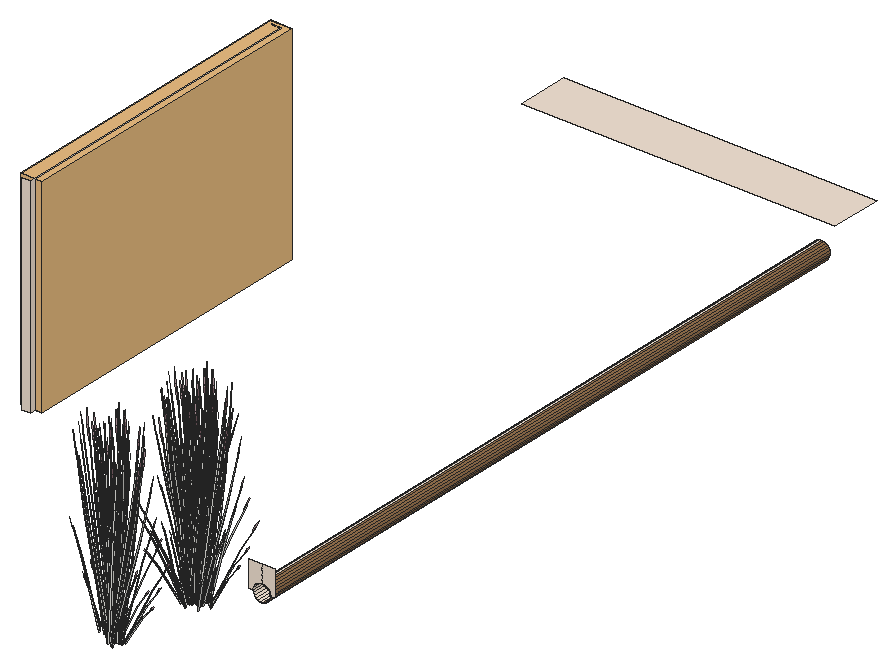
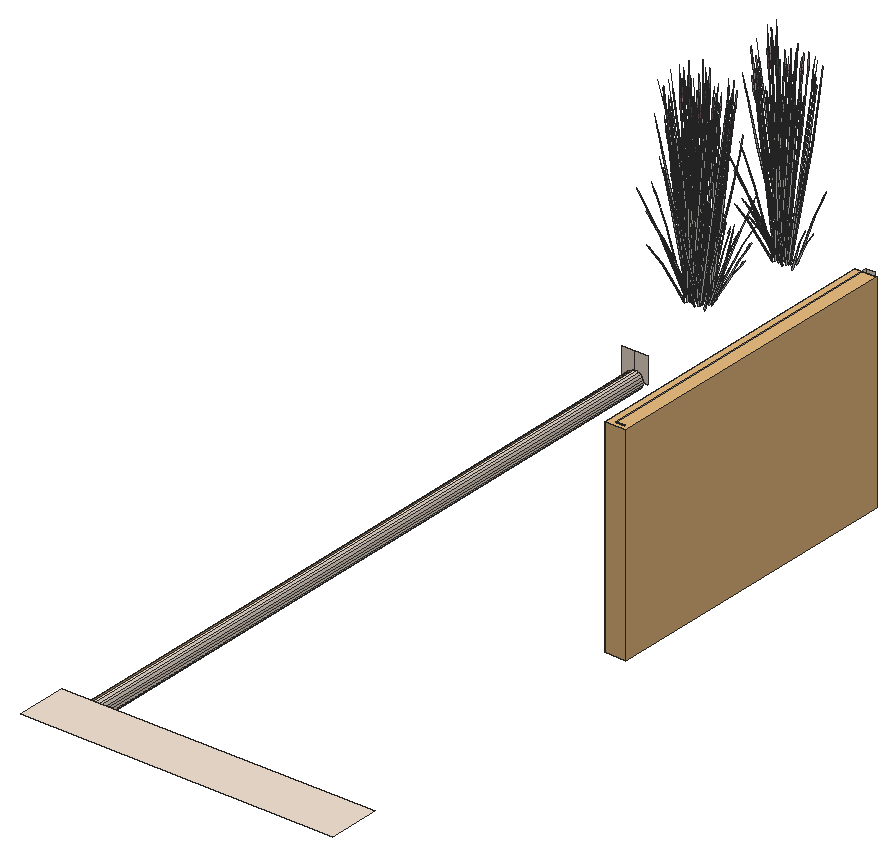
# SketchUp Ruby script. Lengths in inches.
U = 1.inch
M = Sketchup.active_model
def pt(a) = Geom::Point3d.new(a.map { |v| v * U })
def face(e, loops, mat)
  f = e.add_face(loops[0].map { |a| pt(a) })
  loops[1..].each { |l| e.add_face(l.map { |a| pt(a) }).erase! }
  f.material = f.back_material = mat if mat
  f
end
# faces: each face lists its corners as indices into pts; further lists are holes
def faces(e, pts, list, mat = nil) = list.each { |f| face(e, (f[0].is_a?(Array) ? f : [f]).map { |l| l.map { |i| pts[i] } }, mat) }
# xy, xz, yz: faces in a plane at the given z, y or x. An outline is a flat list of corners, or four numbers for a rectangle; further outlines are holes
def ring(l) = l.size == 4 ? [[l[0], l[1]], [l[2], l[1]], [l[2], l[3]], [l[0], l[3]]] : l.each_slice(2).to_a
def flat(e, list, mat, &to3) = list.each { |f| face(e, (f[0].is_a?(Array) ? f : [f]).map { |l| ring(l).map { |u, v| to3.(u, v) } }, mat) }
def xy(e, z, list, mat = nil) = flat(e, list, mat) { |x, y| [x, y, z] }
def xz(e, y, list, mat = nil) = flat(e, list, mat) { |x, z| [x, y, z] }
def yz(e, x, list, mat = nil) = flat(e, list, mat) { |y, z| [x, y, z] }
def lines(e, pts, list) = list.each { |a, b| e.add_line(pt(pts[a]), pt(pts[b])) }
# prism: a flat outline (further loops are holes) pulled along v
def prism(e, loops, v, mat = nil)
  f = face(e, loops, mat); d = Geom::Vector3d.new(v.map { |x| x * U })
  f.pushpull(f.normal.samedirection?(d) ? d.length : -d.length)
end
def box(e, o, s, mat = nil) = prism(e, [[o, [o[0] + s[0], o[1], o[2]], [o[0] + s[0], o[1] + s[1], o[2]], [o[0], o[1] + s[1], o[2]]]], [0, 0, s[2]], mat)
def at(x, y, z, deg = 0) = Geom::Transformation.translation(pt([x, y, z])) * Geom::Transformation.rotation(ORIGIN, Z_AXIS, deg.degrees)
def axes(o, x, y, z) = Geom::Transformation.new([*x, 0, *y, 0, *z, 0, *pt(o).to_a, 1])
def part(name) = M.definitions.add(name)
# library, detail: a bought-in or finely detailed component or shape, given as its bounding box
def library(name, o, s) = part(name).tap { |d| box(d.entities, o, s) }
def detail(e, o, s) = box(e.add_group.entities, o, s)
def put(e, d, t, mat = nil) = e.add_instance(d, t).tap { |i| i.material = mat if mat }
def group(e, t, mat = nil) = e.add_group.tap { |g| g.transformation = t; g.material = mat if mat }.entities
root = M.entities
M.materials.add("C01_Vanilla_Cream").color = [244, 228, 212]
M.materials.add("LightPink_Translucent").color = [144, 107, 117]
M.materials["LightPink_Translucent"].alpha = 0.75
M.materials.add("Wood_Floor_01_1K").color = [146, 111, 76]
c1 = part("blade")
p = [[2.15,0.21,22],[0,0.17,0],[0.09,0.45,0],[2.18,0.31,22],[2.29,0.31,22],[0.38,0.45,0],
  [2.48,0.24,33],[2.49,0.24,33],[2.48,0.22,33]]
faces(c1.entities,p,[[0,1,2,3],[4,5,2,3],[6,3,4,7],[8,0,3,6]])
c2 = part("seeds")
p = [[0.3,-0.1,1.38],[-0.01,-0.03,1.59],[-0.01,-0.03,0.03],[0.14,-0.07,-0.07],[0.29,-0.03,3],[0.15,0.01,3.11]]
faces(c2.entities,p,[[0,1,2,3],[1,0,4,5]],"LightPink_Translucent")
c3 = part("blade with seeds")
put(c3.entities,c1,at(0,0,0))
put(c3.entities,c2,axes([2.4,0.25,30.99],[1.5799,-0.05474,1.17369],[-0.12525,1.92788,0.29478],[-0.07173,-0.02425,1.56792]))
c4 = library("Double casement window",[0,0,0],[5.02,56.42,60])
xy(root,498,[[288,324,290,396],[288,468,360,480]],"C01_Vanilla_Cream")
xz(root,306.76,[[354,492,354,498,357,498,357,494,356.48,493.93,356,493.73,355.59,493.41,355.27,493,355.07,492.52,355,492],[359,492,358.93,492.52,358.73,493,358.41,493.41,358,493.73,357.52,493.93,357,494,357,498,360,498,360,492]],"C01_Vanilla_Cream")
xz(root,324,[[288,498,290,546]],"C01_Vanilla_Cream")
xz(root,396,[[288,498,290,546]],"C01_Vanilla_Cream")
yz(root,290,[[[324,498,396,546],[327,501,358.5,543],[361.5,501,393,543]]],"C01_Vanilla_Cream")
p = [[357,306.76,490],[356.48,306.76,490.07],[356.48,468,490.07],[357,468,490],[357.52,306.76,490.07],[357.52,468,490.07],
  [356,306.76,490.27],[356,468,490.27],[358,306.76,490.27],[358,468,490.27],[355.59,306.76,490.59],[355.59,468,490.59],
  [358.41,306.76,490.59],[358.41,468,490.59],[355.27,306.76,491],[355.27,468,491],[358.73,306.76,491],[358.73,468,491],
  [355.07,306.76,491.48],[355.07,468,491.48],[358.93,306.76,491.48],[358.93,468,491.48],[355,306.76,492],[355,468,492],
  [359,306.76,492],[359,468,492],[355.07,306.76,492.52],[355.07,468,492.52],[358.93,306.76,492.52],[358.93,468,492.52],
  [355.27,306.76,493],[355.27,468,493],[358.73,306.76,493],[358.73,468,493],[355.59,306.76,493.41],[355.59,468,493.41],
  [358.41,306.76,493.41],[358.41,468,493.41],[356,306.76,493.73],[356,468,493.73],[358,306.76,493.73],[358,468,493.73],
  [356.48,306.76,493.93],[356.48,468,493.93],[357.52,306.76,493.93],[357.52,468,493.93],[357,306.76,494],[357,468,494]]
faces(root,p,[[0,1,2,3],[1,6,7,2],[6,10,11,7],[10,14,15,11],[14,18,19,15],[18,22,23,19],[22,26,27,23],[26,30,31,27],
  [30,34,35,31],[34,38,39,35],[38,42,43,39],[42,46,47,43]],"C01_Vanilla_Cream")
faces(root,p,[[4,0,3,5],[8,4,5,9],[12,8,9,13],[16,12,13,17],[20,16,17,21],[24,20,21,25],[28,24,25,29],[32,28,29,33],
  [36,32,33,37],[40,36,37,41],[44,40,41,45],[46,44,45,47]],"Wood_Floor_01_1K")
put(root,c3,axes([353.44,266.61,499.52],[-0.13078,-0.42928,-0.23233],[0.51941,-0.1219,0.23233],[-0.10471,-0.0495,1.0423]))
put(root,c3,axes([354.11,266.59,499.86],[0.59825,-0.13076,0.13232],[0.14773,0.48663,0.26315],[-0.05336,-0.0709,1.20305]))
put(root,c3,axes([355.34,264.75,500],[0.56211,-0.32708,-0.21822],[0.3738,0.46216,-0.37502],[0.13869,0.04694,1.19781]))
put(root,c3,axes([353.3,266.8,499.51],[-0.52105,-0.24633,-0.37238],[0.31144,-0.44171,0],[-0.11867,-0.0561,1.18128]))
put(root,c3,axes([356.76,263.88,499.51],[0.52105,0.24633,-0.37238],[-0.31144,0.44171,0],[0.11867,0.0561,1.18128]))
put(root,c3,axes([355.77,265.28,499.65],[0.62289,0,0],[0,0.51004,0],[0,0,1.33805]))
put(root,c3,axes([354.71,265.93,500],[-0.56211,0.32708,-0.21822],[-0.3738,-0.46216,-0.37502],[-0.13869,-0.04694,1.19781]))
put(root,c3,axes([355.95,264.09,499.86],[-0.59825,0.13076,0.13232],[-0.14773,-0.48663,0.26315],[0.05336,0.0709,1.20305]))
put(root,c3,axes([356.61,264.0625,499.52],[0.13078,0.42928,-0.23233],[-0.51941,0.1219,0.23233],[0.10471,0.0495,1.0423]))
put(root,c3,axes([355.57,265.02,499.79],[-0.70367,-0.1038,0.36899],[0.1432,-0.58624,0.1448],[0.10283,0.05661,1.2811]))
put(root,c3,axes([355.01,266.47,499.65],[-0.18165,-0.42474,0],[0.51872,-0.14874,0],[0,0,1.15778]))
put(root,c3,axes([354.66,266.07,499.96],[-0.1074,0.43968,0.1086],[-0.52474,-0.07632,-0.3101],[-0.0955,-0.04515,0.95058]))
put(root,c3,axes([355.6875,266.41,499.64],[0.5845,-0.16716,-0.14398],[0.20539,0.48152,0.00006],[0.06452,-0.01848,1.30423]))
put(root,c3,axes([355.89,266.61,499.86],[0.16083,-0.48962,0.13232],[0.58854,0.13856,0.26315],[-0.10167,0.00238,1.20305]))
put(root,c3,axes([355.76,265.5,499.66],[0.38863,0.31822,0],[-0.38863,0.31822,0],[0,0,1.2695]))
put(root,c3,axes([356.81,265.36,499.86],[-0.43742,-0.35886,0.13232],[0.44081,-0.34807,0.26315],[-0.04831,0.07329,1.20305]))
put(root,c3,axes([356,264.82,499.54],[0.57914,0.08077,-0.46765],[-0.12221,0.49823,-0.12274],[0.17283,0.06037,1.03225]))
put(root,c3,axes([358.56,265.69,500.07],[-0.34399,0.08133,0.86145],[0.16192,-0.33614,0.63294],[0.18249,0.023,0.18974]))
put(root,c3,axes([354.88,266.66,499.65],[-0.56127,-0.22118,0],[0.27012,-0.45959,0],[0,0,1.2203]))
put(root,c3,axes([355.34,266.07,499.85],[-0.54364,-0.39653,-0.18894],[0.45745,-0.44527,0.41347],[-0.14639,0.04639,1.26162]))
put(root,c3,axes([353.91,266.83,499.86],[0.52105,0.24633,0.37238],[-0.31144,0.44171,0],[-0.11867,-0.0561,1.18128]))
put(root,c3,axes([355.75,265.13,500.04],[0.27012,-0.44393,0.33554],[0.56127,0.21365,-0.16149],[0,0.10233,1.07733]))
put(root,c3,axes([355.65,265.38,499.72],[0,0.56976,-0.04228],[-0.69617,0,0],[0,0.01791,1.34526]))
put(root,c3,axes([355.7,264.98,499.66],[0.33445,0.41351,-0.33554],[-0.50659,0.29119,0.16149],[0.10823,0.05117,1.07733]))
put(root,c3,axes([353.61,267.09,499.78],[-0.34808,0.49367,0],[-0.58235,-0.27531,-0.38706],[-0.13264,-0.0627,1.22783]))
put(root,c3,axes([357.17,265.38,499.86],[0,-0.49266,0.37238],[0.62289,0,0],[0,0.11221,1.18128]))
put(root,c3,axes([355.61,265.75,500.04],[0.60457,-0.03041,0.33554],[0.05467,0.50484,-0.16149],[-0.10823,0.05117,1.07733]))
put(root,c3,axes([355.98,265.23,499.96],[0.51872,-0.14368,0.1086],[0.18165,0.41027,-0.3101],[0,0.09029,0.95058]))
put(root,c3,axes([355.07,265.99,499.66],[-0.60457,0.03041,-0.33554],[-0.05467,-0.50484,0.16149],[-0.10823,0.05117,1.07733]))
put(root,c3,axes([357.91,266.23,499.94],[-0.13408,-0.12117,1.07251],[0.17446,-0.40083,-0.23066],[0.27128,0.0543,0.45856]))
put(root,c3,axes([355.52,266.67,499.65],[0.56127,0.22118,0],[-0.27012,0.45959,0],[0,0,1.31215]))
put(root,c3,axes([355.74,267.16,499.64],[-0.34375,-0.4954,-0.03857],[0.58235,-0.27531,0.38706],[-0.1435,0.04717,1.22723]))
put(root,c3,axes([355.62,265.96,499.96],[0.41131,0.296,0.1086],[-0.34309,0.33395,-0.3101],[-0.0955,0.04515,0.95058]))
put(root,c3,axes([356.05,266.875,499.86],[0.52105,-0.24633,0.37238],[0.31144,0.44171,0],[-0.11867,0.0561,1.18128]))
put(root,c3,axes([355.3125,266.49,499.72],[0.24206,0.56598,-0.04509],[-0.69162,0.19832,0],[0.00845,0.01976,1.2913]))
put(root,c3,axes([355.58,267.1,499.52],[-0.51941,-0.1219,-0.23233],[0.13078,-0.42928,0.23233],[-0.10471,0.0495,1.0423]))
put(root,c3,axes([351.83,266.23,499.94],[0.19348,0.04044,1.07251],[0.1247,0.41309,-0.23066],[-0.26282,0.07733,0.45856]))
put(root,c3,axes([357.59,265.46,499.78],[0.69617,0,0],[0,0.55062,-0.38706],[0,0.12541,1.22783]))
put(root,c3,axes([357.3125,265.74,499.65],[-0.69582,-0.00394,-0.03732],[0,-0.55062,0.37457],[-0.02187,0.12535,1.18764]))
put(root,c3,axes([355.81,265.26,500],[0.62699,0.23507,-0.21822],[-0.3019,0.49615,-0.37502],[0.0197,0.12182,1.19781]))
put(root,c3,axes([351.43,267.09,500.07],[0.23202,-0.22328,0.86145],[0.09155,0.35348,0.63294],[-0.16768,0.06329,0.18974]))
put(root,c3,axes([357.17,265.82,499.52],[-0.38863,0.30738,-0.23233],[-0.38863,-0.30738,0.23233],[0,0.09901,1.0423]))
put(root,c3,axes([355.49,265.85,500],[0.06488,0.56215,-0.21822],[-0.6757,0.03399,-0.37502],[-0.11898,0.07488,1.19781]))
put(root,c3,axes([355.74,265.63,499.66],[-0.27012,0.44393,-0.33554],[-0.56127,-0.21365,0.16149],[0,0.10233,1.07733]))
put(root,c3,axes([355.09,266.28,499.54],[-0.375,0.3703,-0.46765],[-0.46584,-0.33578,-0.12274],[-0.15027,0.09237,1.03225]))
put(root,c3,axes([355.75,266.91,499.75],[0.697,0.16013,0.23067],[-0.17437,0.57237,-0.27369],[-0.11536,0.07164,1.23664]))
put(root,c3,axes([355.7,267.29,499.51],[-0.52105,0.24633,-0.37238],[-0.31144,-0.44171,0],[-0.11867,0.0561,1.18128]))
put(root,c3,axes([357.44,265.83,499.51],[0,0.49266,-0.37238],[-0.62289,0,0],[0,0.11221,1.18128]))
put(root,c3,axes([356.64,266.86,500.07],[-0.31347,-0.14166,0.86145],[0.40476,-0.14393,0.63294],[0.10917,0.12192,0.18974]))
put(root,c3,axes([356.18,267.22,499.78],[0.34808,0.49367,0],[-0.58235,0.27531,-0.38706],[-0.13264,0.0627,1.22783]))
put(root,c3,axes([356.73,267.38,499.12],[0.04056,-0.07113,1.32257],[0.51066,-0.20948,-0.20205],[0.15482,0.10842,0.22528]))
put(root,c3,axes([356.06,265.77,499.57],[0.20414,0.45107,-0.51909],[-0.58805,0.16245,-0.13624],[0.02256,0.15274,1.1458]))
put(root,c3,axes([352.04,267.32,499.12],[0.07468,0.04922,1.32257],[0.12663,0.45605,-0.20205],[-0.16551,0.09725,0.22528]))
put(root,c3,axes([356.69,267.5,500],[-0.35702,-0.01545,0.78795],[0.23577,-0.32816,0.43504],[0.14104,0.11659,0.61808]))
put(root,c3,axes([355.53,266.71,499.94],[0.00982,-0.16331,1.07251],[0.4695,-0.18242,-0.23066],[0.14493,0.19547,0.45856]))
put(root,c3,axes([354.35,267.37,499.12],[0.0901,-0.02681,1.32257],[0.54199,0.14755,-0.20205],[0.01585,0.1663,0.22528]))
put(root,c3,axes([353.1,267.43,500.12],[0.50577,-0.08724,0.04881],[0.11627,0.35148,-0.64728],[-0.03206,0.17792,0.5802]))
put(root,c3,axes([352.98,267.81,499.94],[0.17569,-0.07772,1.07251],[0.43377,0.23434,-0.23066],[-0.12911,0.20277,0.45856]))
put(root,c3,axes([358.96,284.58,499.94],[-0.15825,0.09972,1.07251],[-0.47395,-0.17454,-0.23066],[0.08785,-0.21706,0.45856]))
put(root,c3,axes([356.51,284.39,499.94],[-0.03371,0.16116,1.07251],[-0.49286,0.13491,-0.23066],[-0.11521,-0.20831,0.45856]))
put(root,c3,axes([357.78,284.03,499.12],[-0.09338,0.01775,1.32257],[-0.51641,-0.1998,-0.20205],[0.00867,-0.16666,0.22528]))
put(root,c3,axes([356.11,284.64,499.12],[-0.05393,0.0649,1.32257],[-0.545,0.13993,-0.20205],[-0.13166,-0.12729,0.22528]))
put(root,c3,axes([357.01,286.43,499.57],[-0.22864,-0.5052,-0.52377],[0.65862,-0.18195,-0.13747],[-0.02527,-0.17107,1.15612]))
put(root,c3,axes([360.0625,284.88,499.12],[-0.08333,-0.03881,1.32257],[-0.21404,-0.4336,-0.20205],[0.14439,-0.11767,0.22528]))
put(root,c3,axes([356.91,284.98,499.78],[-0.34808,-0.49367,0],[0.58235,-0.27531,-0.38706],[0.13264,-0.0627,1.22783]))
put(root,c3,axes([357.68,284.38,499.6],[-0.38473,0.28263,-0.02919],[-0.35252,-0.30954,-0.13237],[-0.02482,-0.08771,0.43661]))
put(root,c3,axes([355.66,286.36,499.51],[0,-0.49266,-0.37238],[0.62289,0,0],[0,-0.11221,1.18128]))
put(root,c3,axes([357.39,284.9,499.51],[0.52105,-0.24633,-0.37238],[0.31144,0.44171,0],[0.11867,-0.0561,1.18128]))
put(root,c3,axes([360.48,285.75,499.94],[-0.19889,-0.01459,1.07251],[-0.20376,-0.39145,-0.23066],[0.24434,-0.11074,0.45856]))
put(root,c3,axes([358.01,285.91,499.54],[0.375,-0.3703,-0.46765],[0.46584,0.33578,-0.12274],[0.15027,-0.09237,1.03225]))
put(root,c3,axes([357.35,286.56,499.66],[0.27012,-0.44393,-0.33554],[0.56127,0.21365,0.16149],[0,-0.10233,1.07733]))
put(root,c3,axes([357.6,286.34,500],[-0.06488,-0.56215,-0.21822],[0.6757,-0.03399,-0.37502],[0.11898,-0.07488,1.19781]))
put(root,c3,axes([355.92,286.37,499.52],[0.38863,-0.30738,-0.23233],[0.38863,0.30738,0.23233],[0,-0.09901,1.0423]))
put(root,c3,axes([355.77,284.89,499.6],[-0.1606,0.40228,-0.02919],[-0.4943,-0.12375,-0.13237],[-0.07505,-0.0658,0.43661]))
put(root,c3,axes([357.29,286.93,500],[-0.62699,-0.23507,-0.21822],[0.3019,-0.49615,-0.37502],[-0.0197,-0.12182,1.19781]))
put(root,c3,axes([355.5,286.73,499.78],[-0.69617,0,0],[0,-0.55062,-0.38706],[0,-0.12541,1.22783]))
put(root,c3,axes([355.62,285.75,499.94],[0.1087,0.13716,1.07251],[-0.25048,0.37284,-0.23066],[-0.25719,-0.08912,0.45856]))
put(root,c3,axes([357.51,285.09,499.52],[0.51941,0.1219,-0.23233],[-0.13078,0.42928,0.23233],[0.10471,-0.0495,1.0423]))
put(root,c3,axes([356.04,286.59,499.75],[-0.51786,0.4142,0.23067],[-0.51817,-0.40984,-0.27369],[-0.01808,-0.11762,1.23664]))
put(root,c3,axes([357.6875,286.78,499.82],[0.6273,0.23878,0.18048],[-0.3019,0.49615,0.37502],[0,-0.11437,1.20407]))
put(root,c3,axes([357.44,287.45,499.83],[0.14756,-0.58378,-0.17572],[0.69966,0.10176,0.38453],[-0.12225,-0.08062,1.1733]))
put(root,c3,axes([357.49,286.45,500.04],[-0.60457,0.03041,0.33554],[-0.05467,-0.50484,-0.16149],[0.10823,-0.05117,1.07733]))
put(root,c3,axes([355.92,286.81,499.86],[0,0.49266,0.37238],[-0.62289,0,0],[0,-0.11221,1.18128]))
put(root,c3,axes([359.48,285.1,499.78],[0.34808,-0.49367,0],[0.58235,0.27531,-0.38706],[0.13264,0.0627,1.22783]))
put(root,c3,axes([357.39,287.21,499.66],[-0.33445,-0.41351,-0.33554],[0.50659,-0.29119,0.16149],[-0.10823,-0.05117,1.07733]))
put(root,c3,axes([357.46,286.63,499.77],[0.24206,0.5509,0.34316],[-0.69162,0.19157,0.13466],[0.00845,-0.10123,1.19142]))
put(root,c3,axes([360.85,287.05,499.49],[-0.35858,0.05912,1.06187],[-0.05708,-0.47061,0.06078],[0.25115,-0.07123,0.60425]))
put(root,c3,axes([361.5,286.63,499.7],[-0.34516,-0.31503,-0.04866],[0.37803,-0.28865,-0.22062],[0.10711,-0.02032,0.72768]))
put(root,c3,axes([357.34,287.0625,500.04],[-0.27012,0.44393,0.33554],[-0.56127,-0.21365,-0.16149],[0,-0.10233,1.07733]))
put(root,c3,axes([358.33,286.67,499.65],[0,-0.57005,0],[0.69617,0,0],[0,0,1.34592]))
put(root,c3,axes([359.18,285.36,499.86],[-0.52105,-0.24633,0.37238],[0.31144,-0.44171,0],[0.11867,0.0561,1.18128]))
put(root,c3,axes([357.09,287.37,499.54],[-0.57914,-0.08077,-0.46765],[0.12221,-0.49823,-0.12274],[-0.17283,-0.06037,1.03225]))
put(root,c3,axes([358,286.32,499.77],[-0.46162,0.4471,0.34316],[-0.54842,-0.39467,0.13466],[0.11129,-0.04462,1.19142]))
put(root,c3,axes([358.51,287.12,499.72],[-0.51786,-0.42404,-0.04598],[0.51817,-0.4243,0],[-0.01808,-0.01481,1.31678]))
put(root,c3,axes([357.2,285.58,499.86],[-0.16083,0.48962,0.13232],[-0.58854,-0.13856,0.26315],[0.10167,-0.00238,1.20305]))
put(root,c3,axes([356.96,285.97,499.2],[-0.548,0.19724,0.96696],[-0.17442,-0.56594,0.37572],[0.3365,0.00941,1.09981]))
put(root,c3,axes([358.43,286.125,499.96],[0.1074,-0.43968,0.1086],[0.52474,0.07632,-0.3101],[0.0955,0.04515,0.95058]))
put(root,c3,axes([357.52,287.17,499.77],[0.70367,0.1038,0.34316],[-0.1432,0.58624,0.13466],[-0.10283,-0.05661,1.19142]))
put(root,c3,axes([361.24,286.74,499.12],[-0.0291,-0.0748,1.32257],[0.20181,-0.43752,-0.20205],[0.20357,-0.00629,0.22528]))
put(root,c3,axes([355.23,286.67,499.12],[0.01412,0.07764,1.32257],[-0.28464,0.40547,-0.20205],[-0.20218,-0.02044,0.22528]))
put(root,c3,axes([358.21,286.24,500.04],[-0.33445,-0.41351,0.33554],[0.50659,-0.29119,-0.16149],[0.10823,0.05117,1.07733]))
put(root,c3,axes([356.48,288.13,499.52],[-0.13078,-0.42928,-0.23233],[0.51941,-0.1219,0.23233],[-0.10471,-0.0495,1.0423]))
put(root,c3,axes([357.15,288.1,499.86],[0.59825,-0.13076,0.13232],[0.14773,0.48663,0.26315],[-0.05336,-0.0709,1.20305]))
put(root,c3,axes([358.38,286.27,500],[0.56211,-0.32708,-0.21822],[0.3738,0.46216,-0.37502],[0.13869,0.04694,1.19781]))
put(root,c3,axes([356.33,288.3125,499.51],[-0.52105,-0.24633,-0.37238],[0.31144,-0.44171,0],[-0.11867,-0.0561,1.18128]))
put(root,c3,axes([359.8,285.4,499.51],[0.52105,0.24633,-0.37238],[-0.31144,0.44171,0],[0.11867,0.0561,1.18128]))
put(root,c3,axes([358.81,286.8,499.65],[0.62289,0,0],[0,0.51004,0],[0,0,1.33805]))
put(root,c3,axes([357.75,287.44,500],[-0.56211,0.32708,-0.21822],[-0.3738,-0.46216,-0.37502],[-0.13869,-0.04694,1.19781]))
put(root,c3,axes([358.98,285.61,499.86],[-0.59825,0.13076,0.13232],[-0.14773,-0.48663,0.26315],[0.05336,0.0709,1.20305]))
put(root,c3,axes([359.65,285.58,499.52],[0.13078,0.42928,-0.23233],[-0.51941,0.1219,0.23233],[0.10471,0.0495,1.0423]))
put(root,c3,axes([358.61,286.54,499.79],[-0.70367,-0.1038,0.36899],[0.1432,-0.58624,0.1448],[0.10283,0.05661,1.2811]))
put(root,c3,axes([358.04,287.99,499.65],[-0.18165,-0.42474,0],[0.51872,-0.14874,0],[0,0,1.15778]))
put(root,c3,axes([357.7,287.59,499.96],[-0.1074,0.43968,0.1086],[-0.52474,-0.07632,-0.3101],[-0.0955,-0.04515,0.95058]))
put(root,c3,axes([358.72,287.93,499.64],[0.5845,-0.16716,-0.14398],[0.20539,0.48152,0.00006],[0.06452,-0.01848,1.30423]))
put(root,c3,axes([358.93,288.13,499.86],[0.16083,-0.48962,0.13232],[0.58854,0.13856,0.26315],[-0.10167,0.00238,1.20305]))
put(root,c3,axes([358.79,287.02,499.66],[0.38863,0.31822,0],[-0.38863,0.31822,0],[0,0,1.2695]))
put(root,c3,axes([359.85,286.88,499.86],[-0.43742,-0.35886,0.13232],[0.44081,-0.34807,0.26315],[-0.04831,0.07329,1.20305]))
put(root,c3,axes([359.04,286.34,499.54],[0.57914,0.08077,-0.46765],[-0.12221,0.49823,-0.12274],[0.17283,0.06037,1.03225]))
put(root,c3,axes([357.92,288.18,499.65],[-0.56127,-0.22118,0],[0.27012,-0.45959,0],[0,0,1.2203]))
put(root,c3,axes([358.38,287.59,499.85],[-0.54364,-0.39653,-0.18894],[0.45745,-0.44527,0.41347],[-0.14639,0.04639,1.26162]))
put(root,c3,axes([356.95,288.35,499.86],[0.52105,0.24633,0.37238],[-0.31144,0.44171,0],[-0.11867,-0.0561,1.18128]))
put(root,c3,axes([358.79,286.65,500.04],[0.27012,-0.44393,0.33554],[0.56127,0.21365,-0.16149],[0,0.10233,1.07733]))
put(root,c3,axes([358.68,286.9,499.72],[0,0.56976,-0.04228],[-0.69617,0,0],[0,0.01791,1.34526]))
put(root,c3,axes([358.74,286.5,499.66],[0.33445,0.41351,-0.33554],[-0.50659,0.29119,0.16149],[0.10823,0.05117,1.07733]))
put(root,c3,axes([356.65,288.61,499.78],[-0.34808,0.49367,0],[-0.58235,-0.27531,-0.38706],[-0.13264,-0.0627,1.22783]))
put(root,c3,axes([360.21,286.9,499.86],[0,-0.49266,0.37238],[0.62289,0,0],[0,0.11221,1.18128]))
put(root,c3,axes([358.65,287.26,500.04],[0.60457,-0.03041,0.33554],[0.05467,0.50484,-0.16149],[-0.10823,0.05117,1.07733]))
put(root,c3,axes([359.02,286.75,499.96],[0.51872,-0.14368,0.1086],[0.18165,0.41027,-0.3101],[0,0.09029,0.95058]))
put(root,c3,axes([358.11,287.51,499.66],[-0.60457,0.03041,-0.33554],[-0.05467,-0.50484,0.16149],[-0.10823,0.05117,1.07733]))
put(root,c3,axes([360.95,287.75,499.94],[-0.13408,-0.12117,1.07251],[0.17446,-0.40083,-0.23066],[0.27128,0.0543,0.45856]))
put(root,c3,axes([358.55,288.19,499.65],[0.56127,0.22118,0],[-0.27012,0.45959,0],[0,0,1.31215]))
put(root,c3,axes([358.78,288.68,499.64],[-0.34375,-0.4954,-0.03857],[0.58235,-0.27531,0.38706],[-0.1435,0.04717,1.22723]))
put(root,c3,axes([358.66,287.48,499.96],[0.41131,0.296,0.1086],[-0.34309,0.33395,-0.3101],[-0.0955,0.04515,0.95058]))
put(root,c3,axes([359.09,288.39,499.86],[0.52105,-0.24633,0.37238],[0.31144,0.44171,0],[-0.11867,0.0561,1.18128]))
put(root,c3,axes([358.35,288,499.72],[0.24206,0.56598,-0.04509],[-0.69162,0.19832,0],[0.00845,0.01976,1.2913]))
put(root,c3,axes([358.62,288.62,499.52],[-0.51941,-0.1219,-0.23233],[0.13078,-0.42928,0.23233],[-0.10471,0.0495,1.0423]))
put(root,c3,axes([354.87,287.75,499.94],[0.19348,0.04044,1.07251],[0.1247,0.41309,-0.23066],[-0.26282,0.07733,0.45856]))
put(root,c3,axes([360.63,286.98,499.78],[0.69617,0,0],[0,0.55062,-0.38706],[0,0.12541,1.22783]))
put(root,c3,axes([360.35,287.26,499.65],[-0.69582,-0.00394,-0.03732],[0,-0.55062,0.37457],[-0.02187,0.12535,1.18764]))
put(root,c3,axes([358.84,286.78,500],[0.62699,0.23507,-0.21822],[-0.3019,0.49615,-0.37502],[0.0197,0.12182,1.19781]))
put(root,c3,axes([360.21,287.34,499.52],[-0.38863,0.30738,-0.23233],[-0.38863,-0.30738,0.23233],[0,0.09901,1.0423]))
put(root,c3,axes([358.53,287.37,500],[0.06488,0.56215,-0.21822],[-0.6757,0.03399,-0.37502],[-0.11898,0.07488,1.19781]))
put(root,c3,axes([358.78,287.15,499.66],[-0.27012,0.44393,-0.33554],[-0.56127,-0.21365,0.16149],[0,0.10233,1.07733]))
put(root,c3,axes([358.125,287.8,499.54],[-0.375,0.3703,-0.46765],[-0.46584,-0.33578,-0.12274],[-0.15027,0.09237,1.03225]))
put(root,c3,axes([358.79,288.43,499.75],[0.697,0.16013,0.23067],[-0.17437,0.57237,-0.27369],[-0.11536,0.07164,1.23664]))
put(root,c3,axes([358.74,288.8125,499.51],[-0.52105,0.24633,-0.37238],[-0.31144,-0.44171,0],[-0.11867,0.0561,1.18128]))
put(root,c3,axes([360.47,287.35,499.51],[0,0.49266,-0.37238],[-0.62289,0,0],[0,0.11221,1.18128]))
put(root,c3,axes([359.22,288.74,499.78],[0.34808,0.49367,0],[-0.58235,0.27531,-0.38706],[-0.13264,0.0627,1.22783]))
put(root,c3,axes([359.77,288.9,499.12],[0.04056,-0.07113,1.32257],[0.51066,-0.20948,-0.20205],[0.15482,0.10842,0.22528]))
put(root,c3,axes([359.1,287.29,499.57],[0.20414,0.45107,-0.51909],[-0.58805,0.16245,-0.13624],[0.02256,0.15274,1.1458]))
put(root,c3,axes([355.08,288.84,499.12],[0.07468,0.04922,1.32257],[0.12663,0.45605,-0.20205],[-0.16551,0.09725,0.22528]))
put(root,c3,axes([359.73,289.02,500],[-0.35702,-0.01545,0.78795],[0.23577,-0.32816,0.43504],[0.14104,0.11659,0.61808]))
put(root,c3,axes([358.57,288.22,499.94],[0.00982,-0.16331,1.07251],[0.4695,-0.18242,-0.23066],[0.14493,0.19547,0.45856]))
put(root,c3,axes([357.38,288.89,499.12],[0.0901,-0.02681,1.32257],[0.54199,0.14755,-0.20205],[0.01585,0.1663,0.22528]))
put(root,c3,axes([356.14,288.95,500.12],[0.50577,-0.08724,0.04881],[0.11627,0.35148,-0.64728],[-0.03206,0.17792,0.5802]))
put(root,c3,axes([356.02,289.33,499.94],[0.17569,-0.07772,1.07251],[0.43377,0.23434,-0.23066],[-0.12911,0.20277,0.45856]))
put(root,c4,axes([286.7,325.0625,498.3],[1,0,0],[0,1.27666,0],[0,0,0.79394]))
